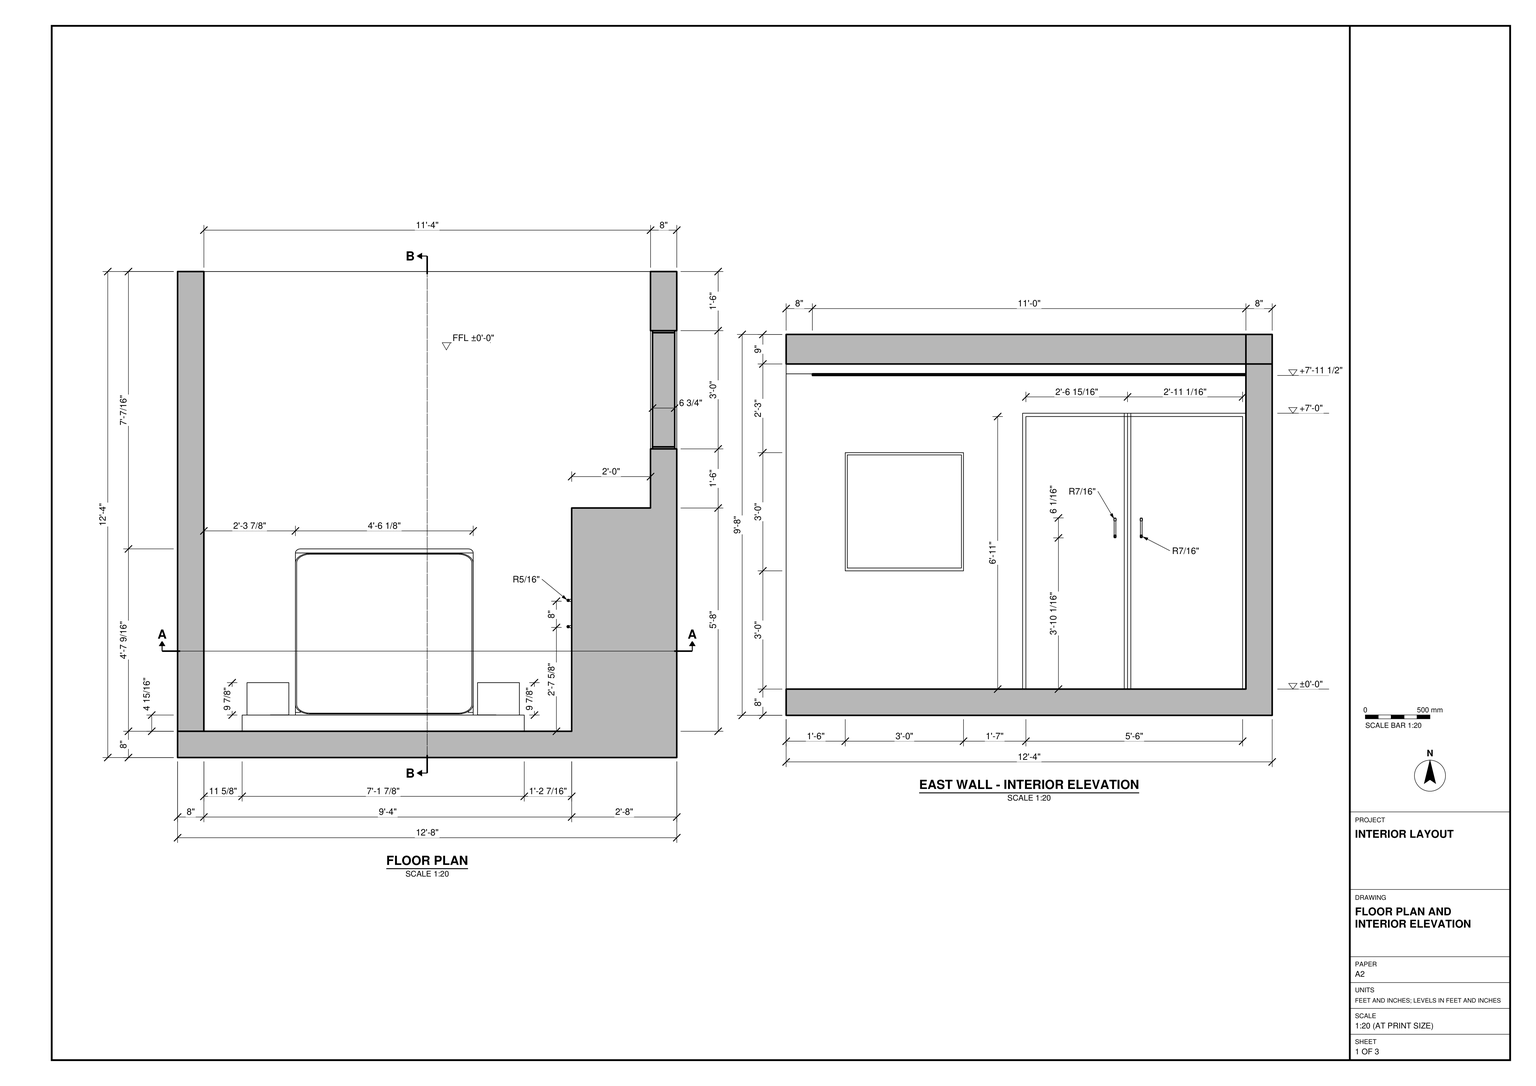
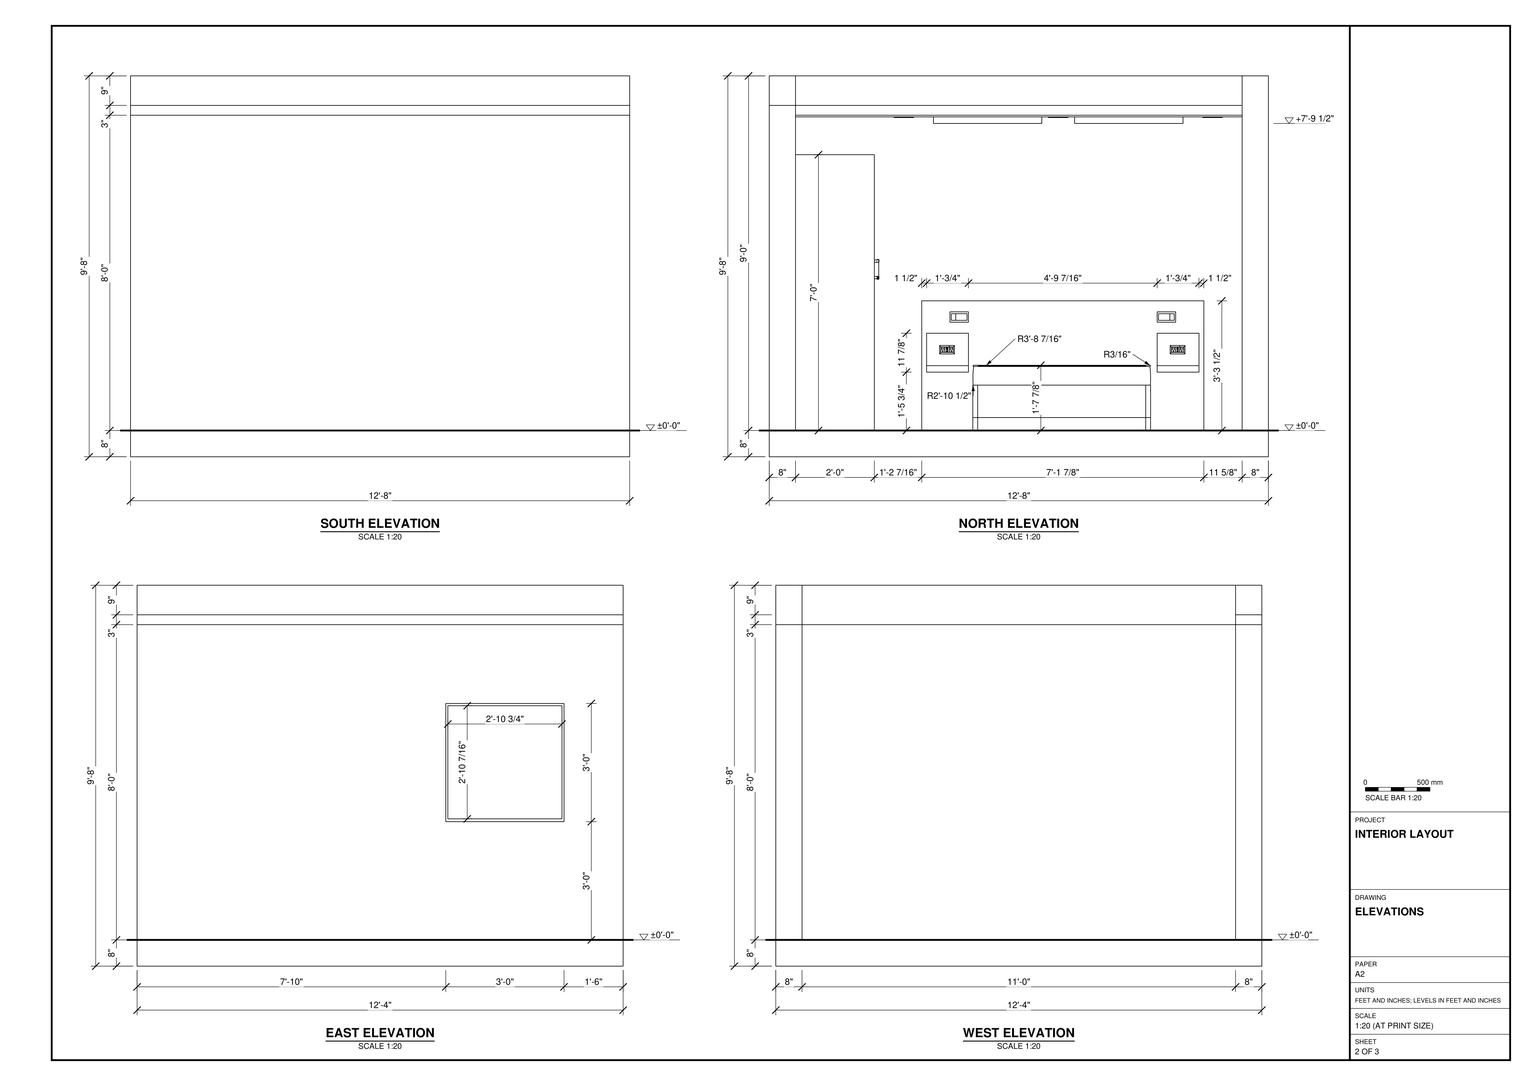
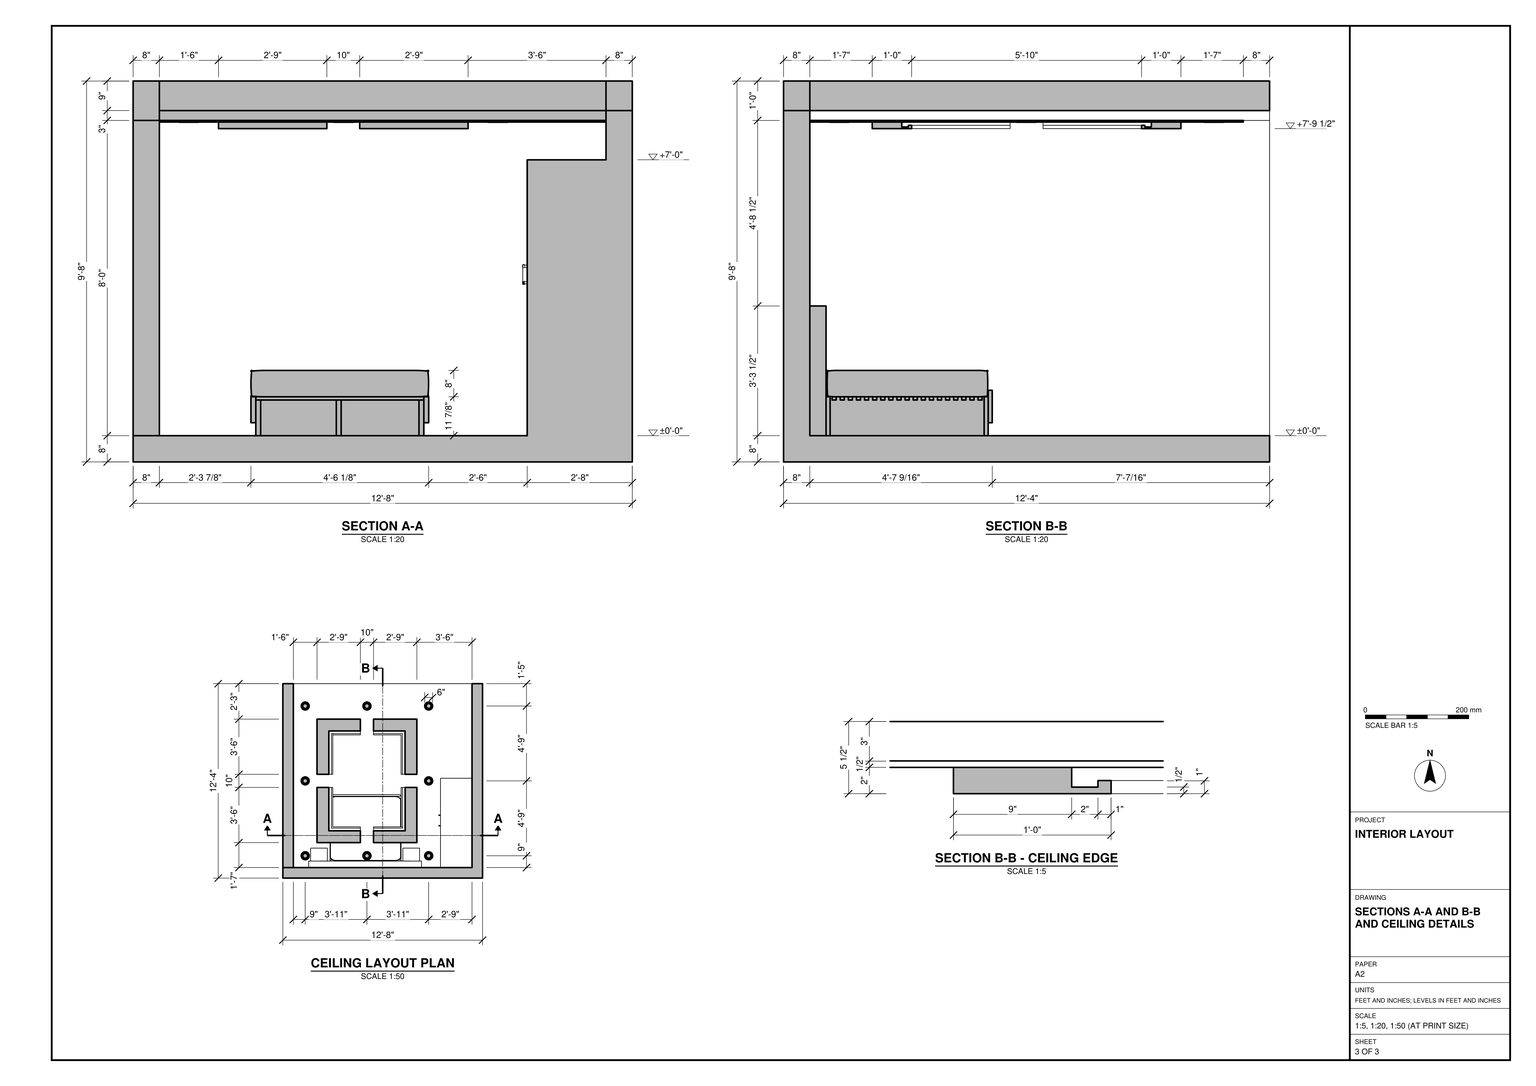
Build the bedroom in SketchUp from task_files/diagram_01.pdf. Work in feet and inches. Set the finished floor at ±0'-0" and make the overall model 12'-8" across the X axis, 12'-4" along the Y axis and 9'-8" high, including the floor and roof slabs.

Follow the floor plan for the south, east and west walls, using the 8" wall thickness shown and leaving the north side open. Fit the square window in the east wall toward the open end. At the other end of that wall, model the built-in wardrobe with its two door fronts and pulls. Place the platform bed with its headboard against the south wall. Use the plan and sections to size the base and mattress, and extend the headboard behind the bedside units on both sides.

Model the ceiling below the flat roof slab. Use the ceiling plan to position the four L-shaped sections and the lights, and use the enlarged edge section for the stepped profile. Decor and loose items may be any suitable library components, for example from 3D Warehouse.

Keep the walls, slabs, ceiling and each furniture or joinery piece as separate groups or components, and use components for repeated parts. Save one SketchUp model as output_files/bedroom_with_built_in_wardrobe_and_stepped_ceiling.skp.

# SketchUp Ruby script. Lengths in inches.
U = 1.inch
M = Sketchup.active_model
def pt(a) = Geom::Point3d.new(a.map { |v| v * U })
def face(e, loops, mat)
  f = e.add_face(loops[0].map { |a| pt(a) })
  loops[1..].each { |l| e.add_face(l.map { |a| pt(a) }).erase! }
  f.material = f.back_material = mat if mat
  f
end
# faces: each face lists its corners as indices into pts; further lists are holes
def faces(e, pts, list, mat = nil) = list.each { |f| face(e, (f[0].is_a?(Array) ? f : [f]).map { |l| l.map { |i| pts[i] } }, mat) }
# xy, xz, yz: faces in a plane at the given z, y or x. An outline is a flat list of corners, or four numbers for a rectangle; further outlines are holes
def ring(l) = l.size == 4 ? [[l[0], l[1]], [l[2], l[1]], [l[2], l[3]], [l[0], l[3]]] : l.each_slice(2).to_a
def flat(e, list, mat, &to3) = list.each { |f| face(e, (f[0].is_a?(Array) ? f : [f]).map { |l| ring(l).map { |u, v| to3.(u, v) } }, mat) }
def xy(e, z, list, mat = nil) = flat(e, list, mat) { |x, y| [x, y, z] }
def xz(e, y, list, mat = nil) = flat(e, list, mat) { |x, z| [x, y, z] }
def yz(e, x, list, mat = nil) = flat(e, list, mat) { |y, z| [x, y, z] }
def lines(e, pts, list) = list.each { |a, b| e.add_line(pt(pts[a]), pt(pts[b])) }
# prism: a flat outline (further loops are holes) pulled along v
def prism(e, loops, v, mat = nil)
  f = face(e, loops, mat); d = Geom::Vector3d.new(v.map { |x| x * U })
  f.pushpull(f.normal.samedirection?(d) ? d.length : -d.length)
end
def box(e, o, s, mat = nil) = prism(e, [[o, [o[0] + s[0], o[1], o[2]], [o[0] + s[0], o[1] + s[1], o[2]], [o[0], o[1] + s[1], o[2]]]], [0, 0, s[2]], mat)
def at(x, y, z, deg = 0) = Geom::Transformation.translation(pt([x, y, z])) * Geom::Transformation.rotation(ORIGIN, Z_AXIS, deg.degrees)
def axes(o, x, y, z) = Geom::Transformation.new([*x, 0, *y, 0, *z, 0, *pt(o).to_a, 1])
def part(name) = M.definitions.add(name)
# library, detail: a bought-in or finely detailed component or shape, given as its bounding box
def library(name, o, s) = part(name).tap { |d| box(d.entities, o, s) }
def detail(e, o, s) = box(e.add_group.entities, o, s)
def put(e, d, t, mat = nil) = e.add_instance(d, t).tap { |i| i.material = mat if mat }
def group(e, t, mat = nil) = e.add_group.tap { |g| g.transformation = t; g.material = mat if mat }.entities
root = M.entities
M.materials.add("[Diamond Stripes]").color = [153, 153, 153]
M.materials.add("[Granite Brown]").color = [126, 104, 91]
M.materials.add("[Mosaic Hexagonal Tile]").color = [168, 194, 223]
M.materials.add("[Sketchy Siding Straight]").color = [235, 219, 175]
M.materials.add("[Translucent_Glass_Blue]").color = [100, 149, 237]
M.materials["[Translucent_Glass_Blue]"].alpha = 0.5
M.materials.add("[Wood Floor Light]").color = [204, 176, 127]
M.materials.add("[Wood Veneer 02]").color = [190, 128, 91]
M.materials.add("[Wood_Bamboo_Medium]").color = [177, 105, 43]
c1 = library("Recessed ceiling light",[0,0,-0.2],[6,6,0.2])
c2 = library("Bed\#1",[-9.84,-88.58,0],[114.17,88.58,39.37])
c3 = library("1-POIGNEE CLC2\#1",[-3.03,-0.375,0],[6.06,0.75,1.42])
c4 = part("Untitled")
xy(c4.entities,34.68,[[46.57,0,194.75,6.75]])
xy(c4.entities,36.94,[[49.13,0,192.19,6.75]],"[Wood_Bamboo_Medium]")
xy(c4.entities,126.69,[[49.13,0,192.19,6.75]],"[Wood_Bamboo_Medium]")
xy(c4.entities,128.49,[[46.57,0,194.75,6.75]],"[Wood_Bamboo_Medium]")
xz(c4.entities,0,[[49.13,36.94,192.19,126.69]],"[Translucent_Glass_Blue]")
xz(c4.entities,0,[[[46.57,34.68,194.75,128.49],[49.13,36.94,192.19,126.69]]],"[Wood_Bamboo_Medium]")
xz(c4.entities,6.75,[[49.13,36.94,192.19,126.69]],"[Translucent_Glass_Blue]")
xz(c4.entities,6.75,[[[46.57,34.68,194.75,128.49],[49.13,36.94,192.19,126.69]]],"[Wood_Bamboo_Medium]")
yz(c4.entities,46.57,[[0,34.68,6.75,128.49]],"[Wood_Bamboo_Medium]")
yz(c4.entities,49.13,[[0,36.94,6.75,126.69]],"[Wood_Bamboo_Medium]")
yz(c4.entities,192.19,[[0,36.94,6.75,126.69]],"[Wood_Bamboo_Medium]")
yz(c4.entities,194.75,[[0,34.68,6.75,128.49]])
xy(root,0,[[0,8,8,140],[0,140,8,148]])
xy(root,96,[[0,8,8,140]])
xy(root,99,[[0,0,0,8,8,8,8,148,152,148,152,0]])
xy(root,108,[[0,0,152,0,152,148,8,148,8,8,0,8],[0,8,8,140],[0,140,8,148]])
xz(root,0,[[0,99,152,108]])
xz(root,8,[[0,0,8,96],[0,96,8,99],[0,99,8,108]])
xz(root,148,[[0,0,8,108],[8,99,152,108]])
yz(root,0,[[8,0,140,96],[140,0,148,96],[8,96,140,108],[140,96,148,108],[0,99,8,108]])
yz(root,8,[[8,96,148,99],[8,99,140,108],[140,99,148,108]])
yz(root,8,[[8,0,148,96]],"[Granite Brown]")
yz(root,152,[[0,99,148,108]])
p = [[90,79,94.51],[91,79,94.51],[91,79,94.01],[93,79,94.01],[93,79,95.51],[69,109,94.51],
  [69,110,94.51],[69,110,94.01],[69,112,94.01],[69,112,95.51],[120,43.05,84],[120,43.05,0],
  [120,45.05,84],[120,45.05,0],[120,44.05,84],[120,44.05,0]]
lines(root,p,[[0,1],[1,2],[2,3],[3,4],[5,6],[6,7],[7,8],[8,9],[10,11],[12,13],[14,15]])
put(root,c1,at(108,14,95.51))
put(root,c1,at(61,14,95.51))
put(root,c1,at(14,14,95.51))
put(root,c1,at(14,71,95.51))
put(root,c1,at(108,71,95.51))
put(root,c1,at(61,128,95.51))
put(root,c1,at(14,128,95.51))
put(root,c1,at(108,128,95.51))
put(root,c2,axes([98.15,8,0],[-0.7524,0,0],[0,-0.627,0],[0,0,1.0032]))
put(root,c3,axes([120,47.86,49.08],[0,0,1],[0,1,0],[-1,0,0]))
put(root,c3,axes([120,39.86,49.08],[0,0,1],[0,1,0],[-1,0,0]))
g1 = group(root,at(8,8,96),"[Diamond Stripes]")
xy(g1,-0.49,[[0,0,136,132]])
xy(g1,0,[[0,0,136,132]])
xz(g1,0,[[0,-0.49,136,0]])
xz(g1,132,[[0,-0.49,136,0]])
yz(g1,136,[[0,-0.49,132,0]])
g2 = group(root,at(26,27,95.51))
xy(g2,-103.51,[[-26,-27,126,121]])
xy(g2,-95.51,[[-26,-19,94,-19,94,49,118,49,118,121,-26,121]],"[Mosaic Hexagonal Tile]")
xy(g2,-59.51,[[118,67,126,103]])
xy(g2,-23.51,[[118,67,126,103]])
xy(g2,-11.51,[[94,-19,118,49]],"[Wood Veneer 02]")
xy(g2,-2,[[0,0,0,42,12,42,12,12,33,12,33,0],[43,0,43,12,64,12,64,42,76,42,76,0],[0,52,0,94,33,94,33,82,12,82,12,52],[64,52,64,82,43,82,43,94,76,94,76,52]],"[Sketchy Siding Straight]")
xy(g2,-1.5,[[9,9,33,9,33,11,11,11,11,42,9,42],[43,9,67,9,67,42,65,42,65,11,43,11],[65,52,67,52,67,85,43,85,43,83,65,83]])
xy(g2,-1.5,[[9,52,11,52,11,83,33,83,33,85,9,85]],"[Sketchy Siding Straight]")
xy(g2,-1,[[11,11,33,11,33,12,12,12,12,42,11,42],[43,11,65,12],[64,12,65,42],[64,52,65,52,65,83,43,83,43,82,64,82]])
xy(g2,-1,[[11,52,12,83],[12,82,33,83]],"[Sketchy Siding Straight]")
xy(g2,0,[[0,0,33,0,33,9,9,9,9,42,0,42],[43,0,76,0,76,42,67.09,42,67.09,9,43,9],[67,52,76,52,76,94,43,94,43,85,67,85]])
xy(g2,0,[[0,52,9,52,9,85,33,85,33,94,0,94]],"[Sketchy Siding Straight]")
xy(g2,12.49,[[-26,-27,126,-27,126,121,118,121,118,-19,-26,-19]])
xz(g2,-27,[[-26,-103.51,126,0.49],[-26,0.49,126,12.49]])
xz(g2,-19,[[-26,0.49,118,12.49]])
xz(g2,-19,[[-26,-95.51,-26,0.49,118,0.49,118,-11.51,94,-11.51,94,-95.51]],"[Granite Brown]")
xz(g2,0,[[0,-2,33,0],[43,-2,76,0]])
xz(g2,9,[[9,-1.5,33,0],[43,-1.5,43,0,67.09,0,67,-1.5]])
xz(g2,11,[[11,-1.5,33,-1],[43,-1.5,65,-1]])
xz(g2,12,[[12,-2,33,-1],[43,-2,64,-1]],"[Sketchy Siding Straight]")
xz(g2,42,[[0,-2,0,0,9,0,9,-1.5,11,-1.5,11,-1,12,-1,12,-2],[64,-2,64,-1,65,-1,65,-1.5,67,-1.5,67.09,0,76,0,76,-2]],"[Sketchy Siding Straight]")
xz(g2,49,[[94,-95.51,118,-11.51]],"[Wood Veneer 02]")
xz(g2,52,[[64,-2,76,-2,76,0,67,0,67,-1.5,65,-1.5,65,-1,64,-1]])
xz(g2,52,[[0,-2,12,-2,12,-1,11,-1,11,-1.5,9,-1.5,9,0,0,0]],"[Sketchy Siding Straight]")
xz(g2,67,[[118,-59.51,126,-23.51]])
xz(g2,82,[[12,-2,33,-1],[43,-2,64,-1]],"[Sketchy Siding Straight]")
xz(g2,83,[[43,-1.5,65,-1]])
xz(g2,83,[[11,-1.5,12,-1],[12,-1.5,33,-1]],"[Sketchy Siding Straight]")
xz(g2,85,[[43,-1.5,67,0]])
xz(g2,85,[[9,-1.5,33,0]],"[Sketchy Siding Straight]")
xz(g2,94,[[0,-2,33,0],[43,-2,76,0]],"[Sketchy Siding Straight]")
xz(g2,103,[[118,-59.51,126,-23.51]])
xz(g2,121,[[-26,-103.51,126,-95.51],[118,-95.51,126,12.49]])
yz(g2,-26,[[-27,-103.51,121,-95.51],[-27,-95.51,-19,0.49],[-27,0.49,-19,12.49]])
yz(g2,0,[[0,-2,42,0]])
yz(g2,0,[[52,-2,94,0]],"[Sketchy Siding Straight]")
yz(g2,9,[[9,-1.5,42,0]])
yz(g2,9,[[52,-1.5,85,0]],"[Sketchy Siding Straight]")
yz(g2,11,[[11,-1.5,42,-1]])
yz(g2,11,[[52,-1.5,83,-1]],"[Sketchy Siding Straight]")
yz(g2,12,[[12,-2,42,-1],[52,-2,82,-1]],"[Sketchy Siding Straight]")
yz(g2,33,[[0,-2,12,-2,12,-1,11,-1,11,-1.5,9,-1.5,9,0,0,0],[82,-2,94,-2,94,0,85,0,85,-1.5,83,-1.5,83,-1,82,-1]],"[Sketchy Siding Straight]")
yz(g2,43,[[0,-2,0,0,9,0,9,-1.5,11,-1.5,11,-1,12,-1,12,-2]])
yz(g2,43,[[82,-2,82,-1,83,-1,83,-1.5,85,-1.5,85,0,94,0,94,-2]],"[Sketchy Siding Straight]")
yz(g2,64,[[12,-2,42,-1],[52,-2,82,-1]],"[Sketchy Siding Straight]")
yz(g2,65,[[11,-1.5,42,-1],[52,-1.5,83,-1]])
yz(g2,67,[[52,-1.5,85,0]])
yz(g2,76,[[0,-2,42,0],[52,-2,94,0]],"[Sketchy Siding Straight]")
yz(g2,94,[[-19,-95.51,49,-11.51]])
yz(g2,118,[[-19,0.49,121,12.49]])
yz(g2,118,[[[49,-95.51,49,-11.51,-19,-11.51,-19,0.49,121,0.49,121,-95.51],[67,-59.51,103,-23.51]]],"[Granite Brown]")
yz(g2,126,[[[-27,-103.51,121,0.49],[67,-59.51,103,-23.51]],[-27,0.49,121,12.49]])
p = [[67.09,42,0],[67,42,-1.5],[67,9,-1.5],[67.09,9,0]]
faces(g2,p,[[0,1,2,3]])
put(g2,c4,axes([125.375,55.6875,-72.82],[0,0.24294,0],[-1,0,0],[0,0,0.38374]))
g3 = group(g2,at(94,48,-95.51),"[Wood Floor Light]")
yz(g3,0,[[-66,0,0,83]])
